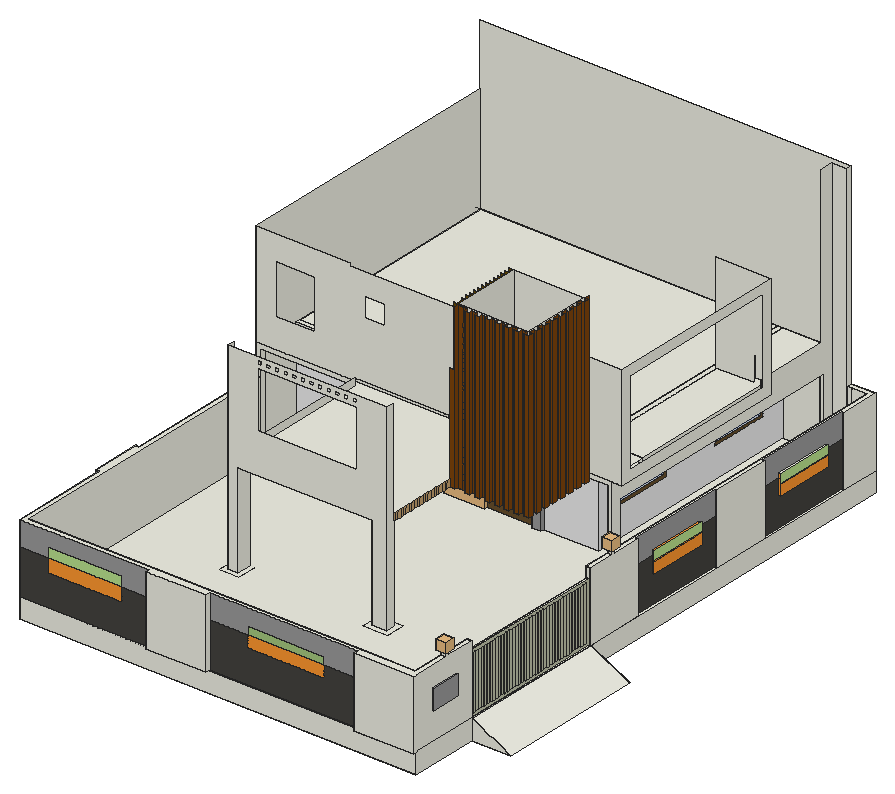
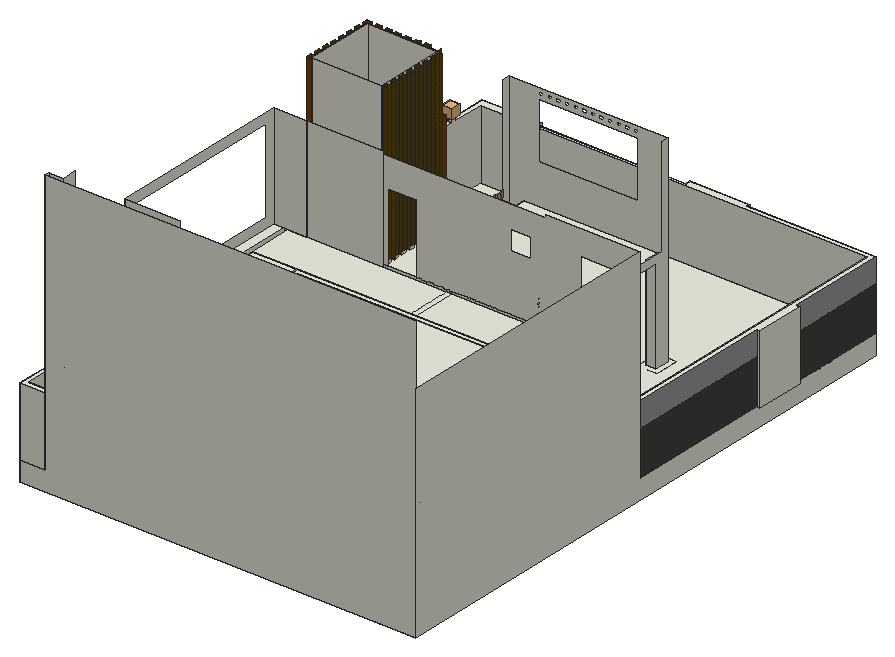
# SketchUp Ruby script. Lengths in inches.
U = 1.inch
M = Sketchup.active_model
def pt(a) = Geom::Point3d.new(a.map { |v| v * U })
def face(e, loops, mat)
  f = e.add_face(loops[0].map { |a| pt(a) })
  loops[1..].each { |l| e.add_face(l.map { |a| pt(a) }).erase! }
  f.material = f.back_material = mat if mat
  f
end
# faces: each face lists its corners as indices into pts; further lists are holes
def faces(e, pts, list, mat = nil) = list.each { |f| face(e, (f[0].is_a?(Array) ? f : [f]).map { |l| l.map { |i| pts[i] } }, mat) }
# xy, xz, yz: faces in a plane at the given z, y or x. An outline is a flat list of corners, or four numbers for a rectangle; further outlines are holes
def ring(l) = l.size == 4 ? [[l[0], l[1]], [l[2], l[1]], [l[2], l[3]], [l[0], l[3]]] : l.each_slice(2).to_a
def flat(e, list, mat, &to3) = list.each { |f| face(e, (f[0].is_a?(Array) ? f : [f]).map { |l| ring(l).map { |u, v| to3.(u, v) } }, mat) }
def xy(e, z, list, mat = nil) = flat(e, list, mat) { |x, y| [x, y, z] }
def xz(e, y, list, mat = nil) = flat(e, list, mat) { |x, z| [x, y, z] }
def yz(e, x, list, mat = nil) = flat(e, list, mat) { |y, z| [x, y, z] }
def lines(e, pts, list) = list.each { |a, b| e.add_line(pt(pts[a]), pt(pts[b])) }
# prism: a flat outline (further loops are holes) pulled along v
def prism(e, loops, v, mat = nil)
  f = face(e, loops, mat); d = Geom::Vector3d.new(v.map { |x| x * U })
  f.pushpull(f.normal.samedirection?(d) ? d.length : -d.length)
end
def box(e, o, s, mat = nil) = prism(e, [[o, [o[0] + s[0], o[1], o[2]], [o[0] + s[0], o[1] + s[1], o[2]], [o[0], o[1] + s[1], o[2]]]], [0, 0, s[2]], mat)
def at(x, y, z, deg = 0) = Geom::Transformation.translation(pt([x, y, z])) * Geom::Transformation.rotation(ORIGIN, Z_AXIS, deg.degrees)
def axes(o, x, y, z) = Geom::Transformation.new([*x, 0, *y, 0, *z, 0, *pt(o).to_a, 1])
def part(name) = M.definitions.add(name)
# library, detail: a bought-in or finely detailed component or shape, given as its bounding box
def library(name, o, s) = part(name).tap { |d| box(d.entities, o, s) }
def detail(e, o, s) = box(e.add_group.entities, o, s)
def put(e, d, t, mat = nil) = e.add_instance(d, t).tap { |i| i.material = mat if mat }
def group(e, t, mat = nil) = e.add_group.tap { |g| g.transformation = t; g.material = mat if mat }.entities
root = M.entities
M.materials.add("C04_Amber_Sunshine").color = [255, 152, 49]
M.materials.add("C08_Toffee_Ember").color = [127, 69, 12]
M.materials.add("D01_Frost_White").color = [238, 238, 227]
M.materials.add("D08_Bronzed_Mustard").color = [102, 74, 0]
M.materials.add("F01_Seafoam_Drift").color = [195, 198, 173]
M.materials.add("Fiber_Insulation_1K").color = [236, 236, 236]
M.materials.add("Glass_Sky Reflection_01").color = [0, 46, 142]
M.materials["Glass_Sky Reflection_01"].alpha = 0.25
M.materials.add("Plywood_08_1K").color = [202, 166, 113]
M.materials.add("Roofing_02_1K").color = [186, 226, 142]
M.materials.add("Roofing_02_1K1").color = [165, 201, 126]
M.materials.add("ThomThom - Waistcoat1").color = [155, 155, 155]
M.materials.add("Wood_Planks_01_1K").color = [69, 67, 63]
M.materials.add("Wood_Veneer_15_1K").color = [103, 79, 44]
c1 = library("porta+4",[0.2,-5.42,1.33],[46.55,4.72,83.21])
c2 = library("Sphere Light",[-6,-6,-6],[12,12,12])
c3 = library("Sphere Light\#1",[-6,-6,-6],[12,12,12])
xy(root,0,[[4,4,484,700],[484,88,532,268]],"D01_Frost_White")
xy(root,24,[[[10,10,478,10,478,694,436,694,436,682,430,682,430,694,376,694,376,415,310,415,310,411,298,411,298,415,136,415,136,411,124,411,124,415,10,415],[298,169,316,181],[124,169,136,187],[430,361,436,373]],[10,421,370,694]],"D01_Frost_White")
xy(root,27,[[196,415,238,421]],"D01_Frost_White")
xy(root,63,[[370,447.97,376,513.97],[370,595,376,661]],"D01_Frost_White")
xy(root,105,[[370,447.97,376,513.97],[370,595,376,661]],"D01_Frost_White")
xy(root,117,[[196,415,238,421]],"D01_Frost_White")
xy(root,120,[[430,373,436,682]],"D01_Frost_White")
xy(root,138,[[136,169,136,187,124,187,124,361,10,361,10,415,124,415,124,411,136,411,136,415,298,415,298,411,310,411,310,415,430,415,430,361,408,361,408,355,412,355,412,349,408,349,408,343,412,343,412,337,408,337,408,331,412,331,412,325,408,325,408,319,412,319,412,313,408,313,408,307,412,307,412,301,408,301,408,295,412,295,412,289,408,289,408,283,412,283,412,277,408,277,408,271,412,271,412,265,406,265,406,269,400,269,400,265,394,265,394,269,388,269,388,265,382,265,382,269,376,269,376,265,370,265,370,269,364,269,364,265,358,265,358,269,352,269,352,265,346,265,346,269,340,269,340,265,334,265,334,269,322,269,322,265,316,265,316,181,298,181,298,169],[124,411,136,415],[298,411,310,415]],"D01_Frost_White")
xy(root,144,[[316,271,320,277],[322,271,406,355],[316,277,320,283],[316,289,320,295],[316,301,320,307],
  [316,313,320,319],[316,325,320,331],[316,337,320,343],[316,349,320,355],[232,361,238,415],
  [238,361,430,415],[436,361,448,586],[10,415,376,415,376,694,370,694,370,421,10,421],[376,415,430,694],[10,421,370,694]],"D01_Frost_White")
xz(root,4,[[4,0,484,24]],"D01_Frost_White")
xz(root,88,[[484,0,532,0,484,24]],"D01_Frost_White")
xz(root,169,[[[124,24,136,24,136,138,298,138,298,24,316,24,316,267,124,267],[160,186,280,255],[264.35,259,269.57,263],[160,259,165.22,263],[253.91,259,259.13,263],[222.61,259,227.83,263],[212.17,259,217.39,263],[201.74,259,206.96,263],[180.87,259,186.09,263],[170.43,259,175.65,263],[274.78,259,280,263],[243.48,259,248.7,263],[233.04,259,238.26,263],[191.3,259,196.52,263]]],"D01_Frost_White")
xz(root,181,[[298,24,316,138]],"D01_Frost_White")
xz(root,187,[[124,24,136,138]],"D01_Frost_White")
xz(root,265,[[316,138,322,267],[334,138,340,336],[346,138,352,336],[358,138,364,336],[370,138,376,336],
  [382,138,388,336],[394,138,400,336],[406,138,412,336]],"C08_Toffee_Ember")
xz(root,268,[[484,0,484,24,532,0]],"D01_Frost_White")
xz(root,269,[[322,138,328,336],[328,138,334,336],[340,138,346,336],[352,138,358,336],[364,138,370,336],
  [376,138,382,336],[388,138,394,336],[400,138,406,336]],"C08_Toffee_Ember")
xz(root,271,[[408,138,412,336]],"C08_Toffee_Ember")
xz(root,271,[[322,144,406,336]],"D01_Frost_White")
xz(root,271,[[316,144,320,336]],"D08_Bronzed_Mustard")
xz(root,277,[[408,138,412,336]],"C08_Toffee_Ember")
xz(root,283,[[408,138,412,336]],"C08_Toffee_Ember")
xz(root,283,[[316,144,320,336]],"D08_Bronzed_Mustard")
xz(root,289,[[408,138,412,336]],"C08_Toffee_Ember")
xz(root,289,[[316,144,320,336]],"D08_Bronzed_Mustard")
xz(root,295,[[408,138,412,336]],"C08_Toffee_Ember")
xz(root,295,[[316,144,320,336]],"D08_Bronzed_Mustard")
xz(root,301,[[408,138,412,336]],"C08_Toffee_Ember")
xz(root,301,[[316,144,320,336]],"D08_Bronzed_Mustard")
xz(root,307,[[408,138,412,336]],"C08_Toffee_Ember")
xz(root,307,[[316,144,320,336]],"D08_Bronzed_Mustard")
xz(root,313,[[408,138,412,336]],"C08_Toffee_Ember")
xz(root,313,[[316,144,320,336]],"D08_Bronzed_Mustard")
xz(root,319,[[408,138,412,336]],"C08_Toffee_Ember")
xz(root,319,[[316,144,320,336]],"D08_Bronzed_Mustard")
xz(root,325,[[408,138,412,336]],"C08_Toffee_Ember")
xz(root,325,[[316,144,320,336]],"D08_Bronzed_Mustard")
xz(root,331,[[408,138,412,336]],"C08_Toffee_Ember")
xz(root,331,[[316,144,320,336]],"D08_Bronzed_Mustard")
xz(root,337,[[408,138,412,336]],"C08_Toffee_Ember")
xz(root,337,[[316,144,320,336]],"D08_Bronzed_Mustard")
xz(root,343,[[408,138,412,336]],"C08_Toffee_Ember")
xz(root,343,[[316,144,320,336]],"D08_Bronzed_Mustard")
xz(root,349,[[408,138,412,336]],"C08_Toffee_Ember")
xz(root,349,[[316,144,320,336]],"D08_Bronzed_Mustard")
xz(root,355,[[408,138,412,336]],"C08_Toffee_Ember")
xz(root,355,[[322,144,406,336]],"D01_Frost_White")
xz(root,355,[[316,144,320,336]],"D08_Bronzed_Mustard")
xz(root,361,[[4,24,10,24,10,138,124,138,124,144,4,144],[430,24,436,24,436,144,408,144,408,138,430,138],[[4,144,124,144,124,147,126,147,126,177,128,177,128,147,274,147,274,231,310,231,310,147,316,147,316,267,118,267,118,270,4,270],[28,180,76,240],[136,216,160,240]],[124,144,232,144,232,147,128,147,128,177,126,177,126,147,124,147],[232,144,238,147],
  [238,144,316,147],[316,144,408,270],[408,144,448,270]],"D01_Frost_White")
xz(root,373,[[430,24,436,120]],"D01_Frost_White")
xz(root,411,[[124,24,136,138],[298,24,310,138]],"ThomThom - Waistcoat1")
xz(root,415,[[[193,24,241,120],[196,27,238,117]],[10,138,376,144],[376,138,430,144]],"D01_Frost_White")
xz(root,415,[[10,24,124,138],[310,24,376,138]],"Fiber_Insulation_1K")
xz(root,415,[[136,24,193,24,193,120,241,120,241,24,298,24,298,138,136,138]],"Wood_Veneer_15_1K")
xz(root,421,[[[10,24,370,144],[196,27,238,117]]],"D01_Frost_White")
xz(root,447.97,[[370,63,376,105]],"D01_Frost_White")
xz(root,513.97,[[370,63,376,105]],"D01_Frost_White")
xz(root,586,[[436,144,436,156,430,156,430,180,427,180,427,150,382,150,382,270,448,270,448,144]],"D01_Frost_White")
xz(root,595,[[370,63,376,105]],"D01_Frost_White")
xz(root,661,[[370,63,376,105]],"D01_Frost_White")
xz(root,682,[[430,24,436,120]],"D01_Frost_White")
xz(root,694,[[10,24,370,144],[376,24,430,144],[436,24,454,344]],"D01_Frost_White")
xz(root,700,[[4,0,4,344,454,344,454,24,484,24,484,0]],"D01_Frost_White")
yz(root,4,[[4,0,4,24,361,24,361,270,700,270,700,0]],"D01_Frost_White")
yz(root,10,[[361,24,367,138],[367,24,415,138],[421,24,694,144]],"D01_Frost_White")
yz(root,124,[[169,24,169,267,178,267,178,147,361,147,361,138,187,138,187,24]],"D01_Frost_White")
yz(root,124,[[411,24,415,138]],"ThomThom - Waistcoat1")
yz(root,136,[[169,24,187,138]],"D01_Frost_White")
yz(root,136,[[411,24,415,138]],"ThomThom - Waistcoat1")
yz(root,196,[[415,27,421,117]],"D01_Frost_White")
yz(root,238,[[415,27,421,117]],"D01_Frost_White")
yz(root,298,[[169,24,181,138]],"D01_Frost_White")
yz(root,298,[[411,24,415,138]],"ThomThom - Waistcoat1")
yz(root,310,[[411,24,415,138]],"ThomThom - Waistcoat1")
yz(root,316,[[169,24,181,24,181,138,178,138,178,267,169,267],[271,144,277,147],[277,144,283,147],[289,144,295,147],[301,144,307,147],
  [313,144,319,147],[325,144,331,147],[337,144,343,147],[349,144,355,147]],"D01_Frost_White")
yz(root,316,[[178,138,182.14,147],[182.14,138,186.29,147],[186.29,138,190.43,147],[190.43,138,194.57,147],[194.57,138,198.71,147],
  [198.71,138,202.86,147],[202.86,138,207,147],[207,138,211.14,147],[211.14,138,215.29,147],[215.29,138,219.43,147],
  [219.43,138,223.57,147],[223.57,138,227.71,147],[227.71,138,231.86,147],[231.86,138,236,147],[236,138,240.14,147],
  [240.14,138,244.29,147],[244.29,138,248.43,147],[248.43,138,252.57,147],[252.57,138,256.71,147],[256.71,138,260.86,147],
  [260.86,138,265,147]],"Plywood_08_1K")
yz(root,320,[[271,144,277,336],[277,144,283,336],[289,144,295,336],[301,144,307,336],[313,144,319,336],
  [325,144,331,336],[337,144,343,336],[349,144,355,336]],"D08_Bronzed_Mustard")
yz(root,322,[[265,138,269,336]],"C08_Toffee_Ember")
yz(root,322,[[271,144,355,336]],"D01_Frost_White")
yz(root,334,[[265,138,269,336]],"C08_Toffee_Ember")
yz(root,340,[[265,138,269,336]],"C08_Toffee_Ember")
yz(root,346,[[265,138,269,336]],"C08_Toffee_Ember")
yz(root,352,[[265,138,269,336]],"C08_Toffee_Ember")
yz(root,358,[[265,138,269,336]],"C08_Toffee_Ember")
yz(root,364,[[265,138,269,336]],"C08_Toffee_Ember")
yz(root,370,[[265,138,269,336]],"C08_Toffee_Ember")
yz(root,370,[[[421,24,694,144],[447.97,63,513.97,105],[595,63,661,105]]],"D01_Frost_White")
yz(root,376,[[265,138,269,336]],"C08_Toffee_Ember")
yz(root,376,[[[415,24,694,144],[444.97,60,516.97,108],[592,60,664,108]]],"Fiber_Insulation_1K")
yz(root,376,[[447.97,63,513.97,105],[595,63,661,105]],"Glass_Sky Reflection_01")
yz(root,376,[[[444.97,60,516.97,108],[447.97,63,513.97,105]],[[592,60,664,108],[595,63,661,105]]],"Wood_Veneer_15_1K")
yz(root,382,[[265,138,269,336]],"C08_Toffee_Ember")
yz(root,388,[[265,138,269,336]],"C08_Toffee_Ember")
yz(root,394,[[265,138,269,336]],"C08_Toffee_Ember")
yz(root,400,[[265,138,269,336]],"C08_Toffee_Ember")
yz(root,406,[[265,138,269,336]],"C08_Toffee_Ember")
yz(root,406,[[271,144,355,336]],"D01_Frost_White")
yz(root,408,[[271,138,277,336],[283,138,289,336],[295,138,301,336],[307,138,313,336],[319,138,325,336],
  [331,138,337,336],[343,138,349,336],[355,138,361,336]],"C08_Toffee_Ember")
yz(root,412,[[265,138,271,336],[277,138,283,336],[289,138,295,336],[301,138,307,336],[313,138,319,336],
  [325,138,331,336],[337,138,343,336],[349,138,355,336]],"C08_Toffee_Ember")
yz(root,430,[[361,24,367,138],[367,24,367,138,415,138,415,144,694,144,694,24,682,24,682,120,373,120,373,24]],"D01_Frost_White")
yz(root,436,[[361,24,373,24,373,120,682,120,682,24,694,24,694,344,676.01,344,676.01,270,676,270,676,156,586,156,586,144,361,144]],"D01_Frost_White")
yz(root,448,[[[361,144,586,270],[373,156,574.02,258]]],"D01_Frost_White")
yz(root,454,[[694,24,700,344]],"D01_Frost_White")
yz(root,484,[[4,0,88,24],[88,0,268,24],[268,0,700,24]],"D01_Frost_White")
p = [[532,268,0],[484,268,24],[484,88,24],[532,88,0],[430,694,144],[430,700,144],
  [10,694,144],[4,694,144],[316,361,144],[316,361,138],[10,367,144],[10,415,144],
  [298,415,24],[298,421,24],[304,187,24],[322,187,24],[322,163,24],[292,163,24],
  [292,181,24],[142,187,24],[142,163,24],[118,163,24],[118,193,24],[130,193,24],
  [484,364,72.67],[484,436,72.67],[484,556,72.67],[484,628,72.67]]
faces(root,p,[[0,1,2,3]],"D01_Frost_White")
lines(root,p,[[4,5],[6,7],[8,9],[10,11],[12,13],[14,15],[15,16],[16,17],[17,18],[19,20],[20,21],[21,22],
  [22,23],[24,25],[26,27]])
put(root,c1,axes([191.83,415.53,22.42],[1.0518,0,0],[0,0.75842,0],[0,0,1.15428]),"D01_Frost_White")
g1 = group(root,at(4,4,24),"D01_Frost_White")
xy(g1,0,[[156,-4,156,0,0,0,0,120,-4,120,-4,180,0,180,0,357,6,357,6,6,474,6,474,84,475,84,475,264,474,264,474,690,450,690,450,696,480,696,480,648,477,648,477,528,480,528,480,456,477,456,477,336,480,336,480,264,478,264,478,84,480,84,480,-4,408,-4,408,2,228,2,228,-4]])
xy(g1,3,[[475,87,478,89.15],[475,91.3,478,93.44],[475,95.59,478,97.74],[475,99.89,478,102.04],[475,104.19,478,106.33],
  [475,108.48,478,110.63],[475,112.78,478,114.93],[475,117.07,478,119.22],[475,121.37,478,123.52],[475,125.67,478,127.81],
  [475,129.96,478,132.11],[475,134.26,478,136.41],[475,138.56,478,140.7],[475,142.85,478,145],[475,147.15,478,149.3],
  [475,151.44,478,153.59],[475,155.74,478,157.89],[475,160.04,478,162.19],[475,164.33,478,166.48],[475,168.63,478,170.78],
  [475,172.93,478,175.07],[475,177.22,478,179.37],[475,181.52,478,183.67],[475,185.81,478,187.96],[475,190.11,478,192.26],
  [475,194.41,478,196.56],[475,198.7,478,200.85],[475,203,478,205.15],[475,207.3,478,209.44],[475,211.59,478,213.74],
  [475,215.89,478,218.04],[475,220.19,478,222.33],[475,224.48,478,226.63],[475,228.78,478,230.93],[475,233.07,478,235.22],
  [475,237.37,478,239.52],[475,241.67,478,243.81],[475,245.96,478,248.11],[475,250.26,478,252.41],[475,254.56,478,256.7],
  [475,258.85,478,261]])
xy(g1,35.375,[[477,360,480,432],[477,552,480,624]],"C04_Amber_Sunshine")
xy(g1,36,[[480,23.37,483,59.37]],"ThomThom - Waistcoat1")
xy(g1,60,[[477,552,480,624]])
xy(g1,60,[[477,360,480,432]],"C04_Amber_Sunshine")
xy(g1,60,[[480,23.37,483,59.37]],"ThomThom - Waistcoat1")
xy(g1,69,[[475,87,478,89.15],[475,91.3,478,93.44],[475,95.59,478,97.74],[475,99.89,478,102.04],[475,104.19,478,106.33],
  [475,108.48,478,110.63],[475,112.78,478,114.93],[475,117.07,478,119.22],[475,121.37,478,123.52],[475,125.67,478,127.81],
  [475,129.96,478,132.11],[475,134.26,478,136.41],[475,138.56,478,140.7],[475,142.85,478,145],[475,147.15,478,149.3],
  [475,151.44,478,153.59],[475,155.74,478,157.89],[475,160.04,478,162.19],[475,164.33,478,166.48],[475,168.63,478,170.78],
  [475,172.93,478,175.07],[475,177.22,478,179.37],[475,181.52,478,183.67],[475,185.81,478,187.96],[475,190.11,478,192.26],
  [475,194.41,478,196.56],[475,198.7,478,200.85],[475,203,478,205.15],[475,207.3,478,209.44],[475,211.59,478,213.74],
  [475,215.89,478,218.04],[475,220.19,478,222.33],[475,224.48,478,226.63],[475,228.78,478,230.93],[475,233.07,478,235.22],
  [475,237.37,478,239.52],[475,241.67,478,243.81],[475,245.96,478,248.11],[475,250.26,478,252.41],[475,254.56,478,256.7],
  [475,258.85,478,261]])
xy(g1,72,[[475,84,478,264]])
xy(g1,84,[[156,-4,228,-4,228,2,408,2,408,-4,480,-4,480,45,474,45,474,6,6,6,6,357,0,357,0,180,-4,180,-4,120,0,120,0,0,156,0],[474,48.71,480,84],[474,264,480,297],[474,300,480,300,480,336,477,336,477,456,480,456,480,528,477,528,477,648,480,648,480,696,450,696,450,690,474,690]])
xy(g1,90,[[474,45,480,48.71],[474,297,477,298.5],[477,297,480,298.5],[474,298.5,477,300],[477,298.5,480,300]])
xz(g1,-4,[[156,0,228,84],[408,0,480,84]])
xz(g1,0,[[33.58,37.94,123.35,54]],"C04_Amber_Sunshine")
xz(g1,0,[[33.58,54,123.35,65.99]],"Roofing_02_1K")
xz(g1,0,[[0,54,33.58,54,33.58,65.99,123.35,65.99,123.35,54,156,54,156,84,0,84]],"ThomThom - Waistcoat1")
xz(g1,0,[[0,0,156,0,156,54,123.35,54,123.35,37.94,33.58,37.94,33.58,54,0,54]],"Wood_Planks_01_1K")
xz(g1,2,[[274.12,39.74,367.08,54]],"C04_Amber_Sunshine")
xz(g1,2,[[274.12,54,367.08,63.5]],"Roofing_02_1K1")
xz(g1,2,[[228,54,274.12,54,274.12,63.5,367.08,63.5,367.08,54,408,54,408,84,228,84]],"ThomThom - Waistcoat1")
xz(g1,2,[[228,0,408,0,408,54,367.08,54,367.08,39.74,274.12,39.74,274.12,54,228,54]],"Wood_Planks_01_1K")
xz(g1,6,[[6,0,426,84],[426,0,474,84]])
xz(g1,23.37,[[480,36,483,60]],"ThomThom - Waistcoat1")
xz(g1,45,[[474,84,480,90]])
xz(g1,48.71,[[474,84,480,90]])
xz(g1,59.37,[[480,36,483,60]],"ThomThom - Waistcoat1")
xz(g1,84,[[474,0,475,84],[478,0,480,84],[475,72,478,84]])
xz(g1,87,[[475,3,478,69]])
xz(g1,89.15,[[475,3,478,69]])
xz(g1,91.3,[[475,3,478,69]])
xz(g1,93.44,[[475,3,478,69]])
xz(g1,95.59,[[475,3,478,69]])
xz(g1,97.74,[[475,3,478,69]])
xz(g1,99.89,[[475,3,478,69]])
xz(g1,102.04,[[475,3,478,69]])
xz(g1,104.19,[[475,3,478,69]])
xz(g1,106.33,[[475,3,478,69]])
xz(g1,108.48,[[475,3,478,69]])
xz(g1,110.63,[[475,3,478,69]])
xz(g1,112.78,[[475,3,478,69]])
xz(g1,114.93,[[475,3,478,69]])
xz(g1,117.07,[[475,3,478,69]])
xz(g1,119.22,[[475,3,478,69]])
xz(g1,120,[[-4,0,0,84]])
xz(g1,121.37,[[475,3,478,69]])
xz(g1,123.52,[[475,3,478,69]])
xz(g1,125.67,[[475,3,478,69]])
xz(g1,127.81,[[475,3,478,69]])
xz(g1,129.96,[[475,3,478,69]])
xz(g1,132.11,[[475,3,478,69]])
xz(g1,134.26,[[475,3,478,69]])
xz(g1,136.41,[[475,3,478,69]])
xz(g1,138.56,[[475,3,478,69]])
xz(g1,140.7,[[475,3,478,69]])
xz(g1,142.85,[[475,3,478,69]])
xz(g1,145,[[475,3,478,69]])
xz(g1,147.15,[[475,3,478,69]])
xz(g1,149.3,[[475,3,478,69]])
xz(g1,151.44,[[475,3,478,69]])
xz(g1,153.59,[[475,3,478,69]])
xz(g1,155.74,[[475,3,478,69]])
xz(g1,157.89,[[475,3,478,69]])
xz(g1,160.04,[[475,3,478,69]])
xz(g1,162.19,[[475,3,478,69]])
xz(g1,164.33,[[475,3,478,69]])
xz(g1,166.48,[[475,3,478,69]])
xz(g1,168.63,[[475,3,478,69]])
xz(g1,170.78,[[475,3,478,69]])
xz(g1,172.93,[[475,3,478,69]])
xz(g1,175.07,[[475,3,478,69]])
xz(g1,177.22,[[475,3,478,69]])
xz(g1,179.37,[[475,3,478,69]])
xz(g1,180,[[-4,0,0,84]])
xz(g1,181.52,[[475,3,478,69]])
xz(g1,183.67,[[475,3,478,69]])
xz(g1,185.81,[[475,3,478,69]])
xz(g1,187.96,[[475,3,478,69]])
xz(g1,190.11,[[475,3,478,69]])
xz(g1,192.26,[[475,3,478,69]])
xz(g1,194.41,[[475,3,478,69]])
xz(g1,196.56,[[475,3,478,69]])
xz(g1,198.7,[[475,3,478,69]])
xz(g1,200.85,[[475,3,478,69]])
xz(g1,203,[[475,3,478,69]])
xz(g1,205.15,[[475,3,478,69]])
xz(g1,207.3,[[475,3,478,69]])
xz(g1,209.44,[[475,3,478,69]])
xz(g1,211.59,[[475,3,478,69]])
xz(g1,213.74,[[475,3,478,69]])
xz(g1,215.89,[[475,3,478,69]])
xz(g1,218.04,[[475,3,478,69]])
xz(g1,220.19,[[475,3,478,69]])
xz(g1,222.33,[[475,3,478,69]])
xz(g1,224.48,[[475,3,478,69]])
xz(g1,226.63,[[475,3,478,69]])
xz(g1,228.78,[[475,3,478,69]])
xz(g1,230.93,[[475,3,478,69]])
xz(g1,233.07,[[475,3,478,69]])
xz(g1,235.22,[[475,3,478,69]])
xz(g1,237.37,[[475,3,478,69]])
xz(g1,239.52,[[475,3,478,69]])
xz(g1,241.67,[[475,3,478,69]])
xz(g1,243.81,[[475,3,478,69]])
xz(g1,245.96,[[475,3,478,69]])
xz(g1,248.11,[[475,3,478,69]])
xz(g1,250.26,[[475,3,478,69]])
xz(g1,252.41,[[475,3,478,69]])
xz(g1,254.56,[[475,3,478,69]])
xz(g1,256.7,[[475,3,478,69]])
xz(g1,258.85,[[475,3,478,69]])
xz(g1,261,[[475,3,478,69]])
xz(g1,264,[[474,0,475,84],[478,0,480,84],[475,72,478,84]])
xz(g1,297,[[474,84,480,90]])
xz(g1,300,[[474,84,480,90]])
xz(g1,336,[[477,0,480,54],[477,54,480,84]])
xz(g1,357,[[0,0,6,84]])
xz(g1,360,[[477,35.375,480,54],[477,54,480,60]],"C04_Amber_Sunshine")
xz(g1,432,[[477,35.375,480,54],[477,54,480,60]],"C04_Amber_Sunshine")
xz(g1,456,[[477,0,480,54],[477,54,480,84]])
xz(g1,528,[[477,0,480,54],[477,54,480,84]])
xz(g1,552,[[477,35.375,480,54],[477,54,480,60]],"C04_Amber_Sunshine")
xz(g1,624,[[477,35.375,480,54],[477,54,480,60]],"C04_Amber_Sunshine")
xz(g1,648,[[477,0,480,54],[477,54,480,84]])
xz(g1,690,[[450,0,456,84],[456,0,474,84]])
xz(g1,696,[[450,0,480,84]])
yz(g1,-4,[[120,0,180,84]])
yz(g1,0,[[0,54,120,84],[180,54,357,84]],"ThomThom - Waistcoat1")
yz(g1,0,[[0,0,120,54],[180,0,357,54]],"Wood_Planks_01_1K")
yz(g1,6,[[6,0,351,84],[351,0,357,84]])
yz(g1,156,[[-4,0,0,84]])
yz(g1,228,[[-4,0,2,84]])
yz(g1,408,[[-4,0,2,84]])
yz(g1,450,[[690,0,696,84]])
yz(g1,474,[[6,0,6,84,45,84,45,90,48.71,90,48.71,84,84,84,84,0],[264,0,264,84,297,84,297,90,300,90,300,84,690,84,690,0]])
yz(g1,475,[[[84,0,264,72],[215.89,3,218.04,69],[220.19,3,222.33,69],[224.48,3,226.63,69],[228.78,3,230.93,69],[233.07,3,235.22,69],[237.37,3,239.52,69],[241.67,3,243.81,69],[245.96,3,248.11,69],[250.26,3,252.41,69],[254.56,3,256.7,69],[87,3,89.15,69],[91.3,3,93.44,69],[95.59,3,97.74,69],[99.89,3,102.04,69],[104.19,3,106.33,69],[108.48,3,110.63,69],[112.78,3,114.93,69],[121.37,3,123.52,69],[125.67,3,127.81,69],[129.96,3,132.11,69],[134.26,3,136.41,69],[138.56,3,140.7,69],[142.85,3,145,69],[147.15,3,149.3,69],[151.44,3,153.59,69],[155.74,3,157.89,69],[160.04,3,162.19,69],[164.33,3,166.48,69],[168.63,3,170.78,69],[172.93,3,175.07,69],[177.22,3,179.37,69],[181.52,3,183.67,69],[185.81,3,187.96,69],[190.11,3,192.26,69],[194.41,3,196.56,69],[198.7,3,200.85,69],[203,3,205.15,69],[207.3,3,209.44,69],[211.59,3,213.74,69],[117.07,3,119.22,69],[258.85,3,261,69]]])
yz(g1,477,[[336,54,360,54,360,60,432,60,432,54,456,54,456,84,336,84],[528,54,552,54,552,60,624,60,624,54,648,54,648,84,528,84]],"ThomThom - Waistcoat1")
yz(g1,477,[[336,0,456,0,456,54,432,54,432,35.375,360,35.375,360,54,336,54],[528,0,648,0,648,54,624,54,624,35.375,552,35.375,552,54,528,54]],"Wood_Planks_01_1K")
yz(g1,478,[[[84,0,264,72],[87,3,261,69]],[89.15,3,91.3,69],[93.44,3,95.59,69],[97.74,3,99.89,69],[102.04,3,104.19,69],
  [106.33,3,108.48,69],[110.63,3,112.78,69],[114.93,3,117.07,69],[119.22,3,121.37,69],[123.52,3,125.67,69],
  [127.81,3,129.96,69],[132.11,3,134.26,69],[136.41,3,138.56,69],[140.7,3,142.85,69],[145,3,147.15,69],
  [149.3,3,151.44,69],[153.59,3,155.74,69],[157.89,3,160.04,69],[162.19,3,164.33,69],[166.48,3,168.63,69],
  [170.78,3,172.93,69],[175.07,3,177.22,69],[179.37,3,181.52,69],[183.67,3,185.81,69],[187.96,3,190.11,69],
  [192.26,3,194.41,69],[196.56,3,198.7,69],[200.85,3,203,69],[205.15,3,207.3,69],[209.44,3,211.59,69],
  [213.74,3,215.89,69],[218.04,3,220.19,69],[222.33,3,224.48,69],[226.63,3,228.78,69],[230.93,3,233.07,69],
  [235.22,3,237.37,69],[239.52,3,241.67,69],[243.81,3,245.96,69],[248.11,3,250.26,69],[252.41,3,254.56,69],
  [256.7,3,258.85,69]],"F01_Seafoam_Drift")
yz(g1,480,[[[-4,0,84,0,84,84,48.71,84,48.71,90,45,90,45,84,-4,84],[23.37,36,59.37,60]],[264,0,336,0,336,84,300,84,300,90,297,90,297,84,264,84],[456,0,528,84],[648,0,696,84]])
yz(g1,480,[[360,35.375,432,49.13],[552,35.375,624,48.67]],"C04_Amber_Sunshine")
yz(g1,480,[[552,48.67,624,60],[360,49.13,432,60]],"Roofing_02_1K")
yz(g1,483,[[23.37,36,59.37,60]],"ThomThom - Waistcoat1")
p = [[477.07,46.7,90],[477.07,46.7,96],[477,298.5,90],[477,298.5,96],[0,120,54],[0,180,54]]
lines(g1,p,[[0,1],[2,3],[4,5]])
put(g1,c2,at(477.07,46.7,96))
put(g1,c3,at(477,298.5,96))
